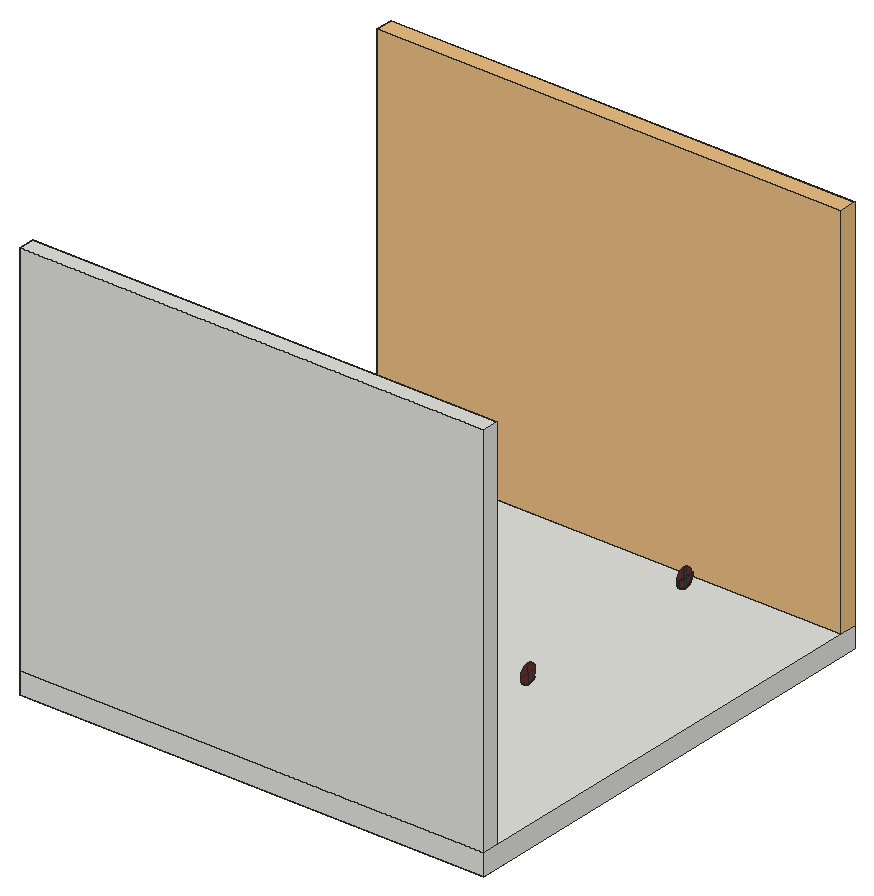
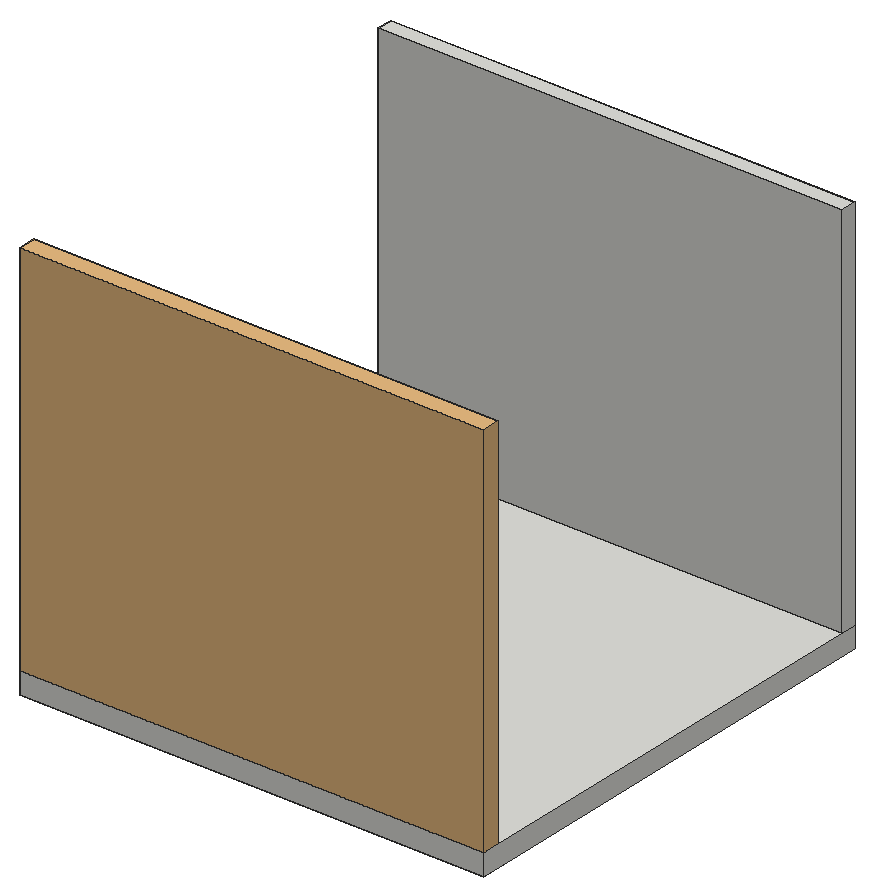
# SketchUp Ruby script. Lengths in millimetres.
U = 1.mm
M = Sketchup.active_model
def pt(a) = Geom::Point3d.new(a.map { |v| v * U })
def face(e, loops, mat)
  f = e.add_face(loops[0].map { |a| pt(a) })
  loops[1..].each { |l| e.add_face(l.map { |a| pt(a) }).erase! }
  f.material = f.back_material = mat if mat
  f
end
# faces: each face lists its corners as indices into pts; further lists are holes
def faces(e, pts, list, mat = nil) = list.each { |f| face(e, (f[0].is_a?(Array) ? f : [f]).map { |l| l.map { |i| pts[i] } }, mat) }
# xy, xz, yz: faces in a plane at the given z, y or x. An outline is a flat list of corners, or four numbers for a rectangle; further outlines are holes
def ring(l) = l.size == 4 ? [[l[0], l[1]], [l[2], l[1]], [l[2], l[3]], [l[0], l[3]]] : l.each_slice(2).to_a
def flat(e, list, mat, &to3) = list.each { |f| face(e, (f[0].is_a?(Array) ? f : [f]).map { |l| ring(l).map { |u, v| to3.(u, v) } }, mat) }
def xy(e, z, list, mat = nil) = flat(e, list, mat) { |x, y| [x, y, z] }
def xz(e, y, list, mat = nil) = flat(e, list, mat) { |x, z| [x, y, z] }
def yz(e, x, list, mat = nil) = flat(e, list, mat) { |y, z| [x, y, z] }
def lines(e, pts, list) = list.each { |a, b| e.add_line(pt(pts[a]), pt(pts[b])) }
# prism: a flat outline (further loops are holes) pulled along v
def prism(e, loops, v, mat = nil)
  f = face(e, loops, mat); d = Geom::Vector3d.new(v.map { |x| x * U })
  f.pushpull(f.normal.samedirection?(d) ? d.length : -d.length)
end
def box(e, o, s, mat = nil) = prism(e, [[o, [o[0] + s[0], o[1], o[2]], [o[0] + s[0], o[1] + s[1], o[2]], [o[0], o[1] + s[1], o[2]]]], [0, 0, s[2]], mat)
def at(x, y, z, deg = 0) = Geom::Transformation.translation(pt([x, y, z])) * Geom::Transformation.rotation(ORIGIN, Z_AXIS, deg.degrees)
def axes(o, x, y, z) = Geom::Transformation.new([*x, 0, *y, 0, *z, 0, *pt(o).to_a, 1])
def part(name) = M.definitions.add(name)
# library, detail: a bought-in or finely detailed component or shape, given as its bounding box
def library(name, o, s) = part(name).tap { |d| box(d.entities, o, s) }
def detail(e, o, s) = box(e.add_group.entities, o, s)
def put(e, d, t, mat = nil) = e.add_instance(d, t).tap { |i| i.material = mat if mat }
def group(e, t, mat = nil) = e.add_group.tap { |g| g.transformation = t; g.material = mat if mat }.entities
root = M.entities
M.materials.add("Uniboard-L17-Ambrette-4K").color = [104, 52, 49]
M.materials.add("Uniboard-L19-Putty-4K").color = [187, 181, 160]
c1 = library("Group\#2",[0,-12,0],[3352.8,126.3,2743.2])
xy(root,413.1,[[2619.9,1332.9,2628.9,1333.4],[2619.9,1336.4,2628.9,1336.9],[2616.9,2747.3,2628.9,2747.8],[2616.9,2750.8,2628.9,2751.3]],"Uniboard-L17-Ambrette-4K")
xy(root,478.1,[[2616.9,2684.3,2628.9,2747.8],[2616.9,2750.8,2628.9,2814.3]],"Uniboard-L17-Ambrette-4K")
xy(root,481.1,[[2616.9,2684.3,2628.9,2747.8],[2616.9,2750.8,2628.9,2814.3]],"Uniboard-L17-Ambrette-4K")
xz(root,2684.3,[[2616.9,476.1,2628.9,478.1],[2616.9,481.1,2628.9,483.1]],"Uniboard-L17-Ambrette-4K")
xz(root,2747.8,[[2616.9,413.1,2628.9,478.1],[2616.9,481.1,2628.9,546.1]],"Uniboard-L17-Ambrette-4K")
xz(root,2750.8,[[2616.9,413.1,2628.9,478.1],[2616.9,481.1,2628.9,546.1]],"Uniboard-L17-Ambrette-4K")
xz(root,2814.3,[[2616.9,476.1,2628.9,478.1],[2616.9,481.1,2628.9,483.1]],"Uniboard-L17-Ambrette-4K")
yz(root,2616.9,[[2747.3,413.1,2745.2,413.2,2741.2,413.6,2739.1,413.9,2733.1,415.1,2731.2,415.7,2729.2,416.3,2727.3,416.9,2725.4,417.7,2723.5,418.4,2721.6,419.3,2718,421.1,2716.2,422.2,2714.5,423.2,2712.8,424.3,2711.1,425.5,2709.5,426.7,2706.3,429.3,2703.3,432.1,2700.5,435.1,2697.9,438.3,2696.7,439.9,2695.5,441.6,2694.4,443.3,2693.4,445,2692.3,446.8,2690.5,450.4,2688.1,456.1,2687.5,458,2686.9,460,2686.3,461.9,2685.1,467.9,2684.8,470,2684.4,474,2684.3,476.1,2684.3,478.1,2747.8,478.1,2747.8,413.1],[2750.8,413.1,2750.8,478.1,2814.3,478.1,2814.3,476.1,2814.2,474,2813.8,470,2813.5,467.9,2813.2,465.9,2812.7,463.9,2812.3,461.9,2811.7,460,2811.1,458,2810.5,456.1,2809.7,454.2,2809,452.3,2808.1,450.4,2806.3,446.8,2805.3,445,2803.1,441.6,2801.9,439.9,2800.7,438.3,2798.1,435.1,2795.3,432.1,2792.3,429.3,2789.1,426.7,2787.5,425.5,2785.8,424.3,2784.1,423.2,2782.4,422.2,2780.6,421.1,2777,419.3,2775.1,418.4,2773.2,417.7,2771.3,416.9,2769.4,416.3,2767.4,415.7,2765.5,415.1,2759.5,413.9,2757.5,413.6,2755.4,413.4,2753.4,413.2,2751.3,413.1],[2684.3,481.1,2684.3,483.1,2684.4,485.2,2684.8,489.2,2685.1,491.3,2686.3,497.3,2686.9,499.2,2687.5,501.2,2688.1,503.1,2690.5,508.8,2692.3,512.4,2693.4,514.2,2694.4,515.9,2695.5,517.6,2696.7,519.3,2697.9,520.9,2700.5,524.1,2703.3,527.1,2706.3,529.9,2709.5,532.5,2711.1,533.7,2712.8,534.9,2714.5,536,2716.2,537,2718,538.1,2721.6,539.9,2723.5,540.8,2725.4,541.5,2727.3,542.3,2729.2,542.9,2731.2,543.5,2733.1,544.1,2739.1,545.3,2741.2,545.6,2745.2,546,2747.3,546.1,2747.8,546.1,2747.8,481.1],[2750.8,481.1,2750.8,546.1,2751.3,546.1,2753.4,546,2755.4,545.8,2757.5,545.6,2759.5,545.3,2765.5,544.1,2767.4,543.5,2769.4,542.9,2771.3,542.3,2773.2,541.5,2775.1,540.8,2777,539.9,2780.6,538.1,2782.4,537,2784.1,536,2785.8,534.9,2787.5,533.7,2789.1,532.5,2792.3,529.9,2795.3,527.1,2798.1,524.1,2800.7,520.9,2801.9,519.3,2803.1,517.6,2805.3,514.2,2806.3,512.4,2808.1,508.8,2809,506.9,2809.7,505,2810.5,503.1,2811.1,501.2,2811.7,499.2,2812.3,497.3,2812.7,495.3,2813.2,493.3,2813.5,491.3,2813.8,489.2,2814.2,485.2,2814.3,483.1,2814.3,481.1]],"Uniboard-L17-Ambrette-4K")
yz(root,2619.9,[[1332.9,413.1,1330.8,413.2,1326.8,413.6,1324.7,413.9,1318.7,415.1,1316.8,415.7,1314.8,416.3,1312.9,416.9,1311,417.7,1309.1,418.4,1307.2,419.3,1303.6,421.1,1301.8,422.2,1300.1,423.2,1298.4,424.3,1296.7,425.5,1295.1,426.7,1291.9,429.3,1288.9,432.1,1286.1,435.1,1283.5,438.3,1282.3,439.9,1281.1,441.6,1280,443.3,1279,445,1277.9,446.8,1276.1,450.4,1273.7,456.1,1273.1,458,1272.5,460,1271.9,461.9,1270.7,467.9,1270.4,470,1270,474,1269.9,476.1,1269.9,478.1,1333.4,478.1,1333.4,413.1],[1336.4,413.1,1336.4,478.1,1399.9,478.1,1399.9,476.1,1399.8,474,1399.4,470,1399.1,467.9,1398.8,465.9,1398.3,463.9,1397.9,461.9,1397.3,460,1396.7,458,1396.1,456.1,1395.3,454.2,1394.6,452.3,1393.7,450.4,1391.9,446.8,1390.9,445,1388.7,441.6,1387.5,439.9,1386.3,438.3,1383.7,435.1,1380.9,432.1,1377.9,429.3,1374.7,426.7,1373.1,425.5,1371.4,424.3,1369.7,423.2,1368,422.2,1366.2,421.1,1362.6,419.3,1360.7,418.4,1358.8,417.7,1356.9,416.9,1355,416.3,1353,415.7,1351.1,415.1,1345.1,413.9,1343.1,413.6,1341,413.4,1339,413.2,1336.9,413.1],[1269.9,481.1,1269.9,483.1,1270,485.2,1270.4,489.2,1270.7,491.3,1271.9,497.3,1272.5,499.2,1273.1,501.2,1273.7,503.1,1276.1,508.8,1277.9,512.4,1279,514.2,1280,515.9,1281.1,517.6,1282.3,519.3,1283.5,520.9,1286.1,524.1,1288.9,527.1,1291.9,529.9,1295.1,532.5,1296.7,533.7,1298.4,534.9,1300.1,536,1301.8,537,1303.6,538.1,1307.2,539.9,1309.1,540.8,1311,541.5,1312.9,542.3,1314.8,542.9,1316.8,543.5,1318.7,544.1,1324.7,545.3,1326.8,545.6,1330.8,546,1332.9,546.1,1333.4,546.1,1333.4,481.1],[1336.4,481.1,1336.4,546.1,1336.9,546.1,1339,546,1341,545.8,1343.1,545.6,1345.1,545.3,1351.1,544.1,1353,543.5,1355,542.9,1356.9,542.3,1358.8,541.5,1360.7,540.8,1362.6,539.9,1366.2,538.1,1368,537,1369.7,536,1371.4,534.9,1373.1,533.7,1374.7,532.5,1377.9,529.9,1380.9,527.1,1383.7,524.1,1386.3,520.9,1387.5,519.3,1388.7,517.6,1390.9,514.2,1391.9,512.4,1393.7,508.8,1394.6,506.9,1395.3,505,1396.1,503.1,1396.7,501.2,1397.3,499.2,1397.9,497.3,1398.3,495.3,1398.8,493.3,1399.1,491.3,1399.4,489.2,1399.8,485.2,1399.9,483.1,1399.9,481.1]],"Uniboard-L17-Ambrette-4K")
p = [[2628.9,1332.9,413.1],[2628.9,1330.8,413.2],[2619.9,1330.8,413.2],[2619.9,1332.9,413.1],[2628.9,1339,413.2],[2628.9,1336.9,413.1],
  [2619.9,1336.9,413.1],[2619.9,1339,413.2],[2628.9,2747.3,413.1],[2628.9,2745.2,413.2],[2616.9,2745.2,413.2],[2616.9,2747.3,413.1],
  [2628.9,2753.4,413.2],[2628.9,2751.3,413.1],[2616.9,2751.3,413.1],[2616.9,2753.4,413.2],[2628.9,1328.8,413.4],[2619.9,1328.8,413.4],
  [2628.9,1341,413.4],[2619.9,1341,413.4],[2628.9,2743.2,413.4],[2616.9,2743.2,413.4],[2628.9,2755.4,413.4],[2616.9,2755.4,413.4],
  [2628.9,1326.8,413.6],[2619.9,1326.8,413.6],[2628.9,1343.1,413.6],[2619.9,1343.1,413.6],[2628.9,2741.2,413.6],[2616.9,2741.2,413.6],
  [2628.9,2757.5,413.6],[2616.9,2757.5,413.6],[2628.9,1324.7,413.9],[2619.9,1324.7,413.9],[2628.9,1345.1,413.9],[2619.9,1345.1,413.9],
  [2628.9,2739.1,413.9],[2616.9,2739.1,413.9],[2628.9,2759.5,413.9],[2616.9,2759.5,413.9],[2628.9,1322.7,414.3],[2619.9,1322.7,414.3],
  [2628.9,1347.1,414.3],[2619.9,1347.1,414.3],[2628.9,2737.1,414.3],[2616.9,2737.1,414.3],[2628.9,2761.5,414.3],[2616.9,2761.5,414.3],
  [2628.9,1320.7,414.7],[2619.9,1320.7,414.7],[2628.9,1349.1,414.7],[2619.9,1349.1,414.7],[2628.9,2735.1,414.7],[2616.9,2735.1,414.7],
  [2628.9,2763.5,414.7],[2616.9,2763.5,414.7],[2628.9,1318.7,415.1],[2619.9,1318.7,415.1],[2628.9,1351.1,415.1],[2619.9,1351.1,415.1],
  [2628.9,2733.1,415.1],[2616.9,2733.1,415.1],[2628.9,2765.5,415.1],[2616.9,2765.5,415.1],[2628.9,1316.8,415.7],[2619.9,1316.8,415.7],
  [2628.9,1353,415.7],[2619.9,1353,415.7],[2628.9,2731.2,415.7],[2616.9,2731.2,415.7],[2628.9,2767.4,415.7],[2616.9,2767.4,415.7],
  [2628.9,1314.8,416.3],[2619.9,1314.8,416.3],[2628.9,1355,416.3],[2619.9,1355,416.3],[2628.9,2729.2,416.3],[2616.9,2729.2,416.3],
  [2628.9,2769.4,416.3],[2616.9,2769.4,416.3],[2628.9,1312.9,416.9],[2619.9,1312.9,416.9],[2628.9,1356.9,416.9],[2619.9,1356.9,416.9],
  [2628.9,2727.3,416.9],[2616.9,2727.3,416.9],[2628.9,2771.3,416.9],[2616.9,2771.3,416.9],[2628.9,1311,417.7],[2619.9,1311,417.7],
  [2628.9,1358.8,417.7],[2619.9,1358.8,417.7],[2628.9,2725.4,417.7],[2616.9,2725.4,417.7],[2628.9,2773.2,417.7],[2616.9,2773.2,417.7],
  [2628.9,1309.1,418.4],[2619.9,1309.1,418.4],[2628.9,1360.7,418.4],[2619.9,1360.7,418.4],[2628.9,2723.5,418.4],[2616.9,2723.5,418.4],
  [2628.9,2775.1,418.4],[2616.9,2775.1,418.4],[2628.9,1307.2,419.3],[2619.9,1307.2,419.3],[2628.9,1362.6,419.3],[2619.9,1362.6,419.3],
  [2628.9,2721.6,419.3],[2616.9,2721.6,419.3],[2628.9,2777,419.3],[2616.9,2777,419.3],[2628.9,1305.4,420.2],[2619.9,1305.4,420.2],
  [2628.9,1364.4,420.2],[2619.9,1364.4,420.2],[2628.9,2719.8,420.2],[2616.9,2719.8,420.2],[2628.9,2778.8,420.2],[2616.9,2778.8,420.2],
  [2628.9,1303.6,421.1],[2619.9,1303.6,421.1],[2628.9,1366.2,421.1],[2619.9,1366.2,421.1],[2628.9,2718,421.1],[2616.9,2718,421.1],
  [2628.9,2780.6,421.1],[2616.9,2780.6,421.1],[2628.9,1301.8,422.2],[2619.9,1301.8,422.2],[2628.9,1368,422.2],[2619.9,1368,422.2],
  [2628.9,2716.2,422.2],[2616.9,2716.2,422.2],[2628.9,2782.4,422.2],[2616.9,2782.4,422.2],[2628.9,1300.1,423.2],[2619.9,1300.1,423.2],
  [2628.9,1369.7,423.2],[2619.9,1369.7,423.2],[2628.9,2714.5,423.2],[2616.9,2714.5,423.2],[2628.9,2784.1,423.2],[2616.9,2784.1,423.2],
  [2628.9,1298.4,424.3],[2619.9,1298.4,424.3],[2628.9,1371.4,424.3],[2619.9,1371.4,424.3],[2628.9,2712.8,424.3],[2616.9,2712.8,424.3],
  [2628.9,2785.8,424.3],[2616.9,2785.8,424.3],[2628.9,1296.7,425.5],[2619.9,1296.7,425.5],[2628.9,1373.1,425.5],[2619.9,1373.1,425.5],
  [2628.9,2711.1,425.5],[2616.9,2711.1,425.5],[2628.9,2787.5,425.5],[2616.9,2787.5,425.5],[2628.9,1295.1,426.7],[2619.9,1295.1,426.7],
  [2628.9,1374.7,426.7],[2619.9,1374.7,426.7],[2628.9,2709.5,426.7],[2616.9,2709.5,426.7],[2628.9,2789.1,426.7],[2616.9,2789.1,426.7],
  [2628.9,1293.5,428],[2619.9,1293.5,428],[2628.9,1376.3,428],[2619.9,1376.3,428],[2628.9,2707.9,428],[2616.9,2707.9,428],
  [2628.9,2790.7,428],[2616.9,2790.7,428],[2628.9,1291.9,429.3],[2619.9,1291.9,429.3],[2628.9,1377.9,429.3],[2619.9,1377.9,429.3],
  [2628.9,2706.3,429.3],[2616.9,2706.3,429.3],[2628.9,2792.3,429.3],[2616.9,2792.3,429.3],[2628.9,1290.4,430.7],[2619.9,1290.4,430.7],
  [2628.9,1379.4,430.7],[2619.9,1379.4,430.7],[2628.9,2704.8,430.7],[2616.9,2704.8,430.7],[2628.9,2793.8,430.7],[2616.9,2793.8,430.7],
  [2628.9,1288.9,432.1],[2619.9,1288.9,432.1],[2628.9,1380.9,432.1],[2619.9,1380.9,432.1],[2628.9,2703.3,432.1],[2616.9,2703.3,432.1],
  [2628.9,2795.3,432.1],[2616.9,2795.3,432.1],[2628.9,1287.5,433.6],[2619.9,1287.5,433.6],[2628.9,1382.3,433.6],[2619.9,1382.3,433.6],
  [2628.9,2701.9,433.6],[2616.9,2701.9,433.6],[2628.9,2796.7,433.6],[2616.9,2796.7,433.6],[2628.9,1286.1,435.1],[2619.9,1286.1,435.1],
  [2628.9,1383.7,435.1],[2619.9,1383.7,435.1],[2628.9,2700.5,435.1],[2616.9,2700.5,435.1],[2628.9,2798.1,435.1],[2616.9,2798.1,435.1],
  [2628.9,1284.8,436.7],[2619.9,1284.8,436.7],[2628.9,1385,436.7],[2619.9,1385,436.7],[2628.9,2699.2,436.7],[2616.9,2699.2,436.7],
  [2628.9,2799.4,436.7],[2616.9,2799.4,436.7],[2628.9,1283.5,438.3],[2619.9,1283.5,438.3],[2628.9,1386.3,438.3],[2619.9,1386.3,438.3],
  [2628.9,2697.9,438.3],[2616.9,2697.9,438.3],[2628.9,2800.7,438.3],[2616.9,2800.7,438.3],[2628.9,2696.7,439.9],[2616.9,2696.7,439.9],
  [2628.9,2801.9,439.9],[2616.9,2801.9,439.9],[2628.9,2695.5,441.6],[2616.9,2695.5,441.6],[2628.9,2803.1,441.6],[2616.9,2803.1,441.6],
  [2628.9,2694.4,443.3],[2616.9,2694.4,443.3],[2628.9,2804.2,443.3],[2616.9,2804.2,443.3],[2628.9,2693.4,445],[2616.9,2693.4,445],
  [2628.9,2805.3,445],[2616.9,2805.3,445],[2628.9,2692.3,446.8],[2616.9,2692.3,446.8],[2628.9,2806.3,446.8],[2616.9,2806.3,446.8],
  [2628.9,2691.4,448.6],[2616.9,2691.4,448.6],[2628.9,2807.2,448.6],[2616.9,2807.2,448.6],[2628.9,2690.5,450.4],[2616.9,2690.5,450.4],
  [2628.9,2808.1,450.4],[2616.9,2808.1,450.4],[2628.9,2689.7,452.3],[2616.9,2689.7,452.3],[2628.9,2809,452.3],[2616.9,2809,452.3],
  [2628.9,2688.9,454.2],[2616.9,2688.9,454.2],[2628.9,2809.7,454.2],[2616.9,2809.7,454.2],[2628.9,2688.1,456.1],[2616.9,2688.1,456.1],
  [2628.9,2810.5,456.1],[2616.9,2810.5,456.1],[2628.9,2687.5,458],[2616.9,2687.5,458],[2628.9,2811.1,458],[2616.9,2811.1,458],
  [2628.9,2686.9,460],[2616.9,2686.9,460],[2628.9,2811.7,460],[2616.9,2811.7,460],[2628.9,2686.3,461.9],[2616.9,2686.3,461.9],
  [2628.9,2812.3,461.9],[2616.9,2812.3,461.9],[2628.9,2685.9,463.9],[2616.9,2685.9,463.9],[2628.9,2812.7,463.9],[2616.9,2812.7,463.9],
  [2628.9,2685.5,465.9],[2616.9,2685.5,465.9],[2628.9,2813.2,465.9],[2616.9,2813.2,465.9],[2628.9,2685.1,467.9],[2616.9,2685.1,467.9],
  [2628.9,2813.5,467.9],[2616.9,2813.5,467.9],[2628.9,2684.8,470],[2616.9,2684.8,470],[2628.9,2813.8,470],[2616.9,2813.8,470],
  [2628.9,2684.6,472],[2616.9,2684.6,472],[2628.9,2814,472],[2616.9,2814,472],[2628.9,2684.4,474],[2616.9,2684.4,474],
  [2628.9,2814.2,474],[2616.9,2814.2,474],[2628.9,2684.3,476.1],[2616.9,2684.3,476.1],[2628.9,2814.3,476.1],[2616.9,2814.3,476.1],
  [2628.9,2684.3,483.1],[2628.9,2684.4,485.2],[2616.9,2684.4,485.2],[2616.9,2684.3,483.1],[2628.9,2814.2,485.2],[2628.9,2814.3,483.1],
  [2616.9,2814.3,483.1],[2616.9,2814.2,485.2],[2628.9,2684.6,487.2],[2616.9,2684.6,487.2],[2628.9,2814,487.2],[2616.9,2814,487.2],
  [2628.9,2684.8,489.2],[2616.9,2684.8,489.2],[2628.9,2813.8,489.2],[2616.9,2813.8,489.2]]
faces(root,p,[[0,1,2,3],[4,5,6,7],[8,9,10,11],[12,13,14,15],[1,16,17,2],[18,4,7,19],[9,20,21,10],[22,12,15,23],
  [16,24,25,17],[26,18,19,27],[20,28,29,21],[30,22,23,31],[24,32,33,25],[34,26,27,35],[28,36,37,29],[38,30,31,39],
  [32,40,41,33],[42,34,35,43],[36,44,45,37],[46,38,39,47],[40,48,49,41],[50,42,43,51],[44,52,53,45],[54,46,47,55],
  [48,56,57,49],[58,50,51,59],[52,60,61,53],[62,54,55,63],[56,64,65,57],[66,58,59,67],[60,68,69,61],[70,62,63,71],
  [64,72,73,65],[74,66,67,75],[68,76,77,69],[78,70,71,79],[72,80,81,73],[82,74,75,83],[76,84,85,77],[86,78,79,87],
  [80,88,89,81],[90,82,83,91],[84,92,93,85],[94,86,87,95],[88,96,97,89],[98,90,91,99],[92,100,101,93],[102,94,95,103],
  [96,104,105,97],[106,98,99,107],[100,108,109,101],[110,102,103,111],[104,112,113,105],[114,106,107,115],[108,116,117,109],[118,110,111,119],
  [112,120,121,113],[122,114,115,123],[116,124,125,117],[126,118,119,127],[120,128,129,121],[130,122,123,131],[124,132,133,125],[134,126,127,135],
  [128,136,137,129],[138,130,131,139],[132,140,141,133],[142,134,135,143],[136,144,145,137],[146,138,139,147],[140,148,149,141],[150,142,143,151],
  [144,152,153,145],[154,146,147,155],[148,156,157,149],[158,150,151,159],[152,160,161,153],[162,154,155,163],[156,164,165,157],[166,158,159,167],
  [160,168,169,161],[170,162,163,171],[164,172,173,165],[174,166,167,175],[168,176,177,169],[178,170,171,179],[172,180,181,173],[182,174,175,183],
  [176,184,185,177],[186,178,179,187],[180,188,189,181],[190,182,183,191],[184,192,193,185],[194,186,187,195],[188,196,197,189],[198,190,191,199],
  [192,200,201,193],[202,194,195,203],[196,204,205,197],[206,198,199,207],[200,208,209,201],[210,202,203,211],[204,212,213,205],[214,206,207,215],
  [208,216,217,209],[218,210,211,219],[212,220,221,213],[222,214,215,223],[216,224,225,217],[226,218,219,227],[220,228,229,221],[230,222,223,231],
  [228,232,233,229],[234,230,231,235],[232,236,237,233],[238,234,235,239],[236,240,241,237],[242,238,239,243],[240,244,245,241],[246,242,243,247],
  [244,248,249,245],[250,246,247,251],[248,252,253,249],[254,250,251,255],[252,256,257,253],[258,254,255,259],[256,260,261,257],[262,258,259,263],
  [260,264,265,261],[266,262,263,267],[264,268,269,265],[270,266,267,271],[268,272,273,269],[274,270,271,275],[272,276,277,273],[278,274,275,279],
  [276,280,281,277],[282,278,279,283],[280,284,285,281],[286,282,283,287],[284,288,289,285],[290,286,287,291],[288,292,293,289],[294,290,291,295],
  [292,296,297,293],[298,294,295,299],[296,300,301,297],[302,298,299,303],[300,304,305,301],[306,302,303,307],[304,308,309,305],[310,306,307,311],
  [312,313,314,315],[316,317,318,319],[313,320,321,314],[322,316,319,323],[320,324,325,321],[326,322,323,327]],"Uniboard-L17-Ambrette-4K")
g1 = group(root,at(0,20.3,0))
box(g1,[0,0,0],[3352.8,3352.8,152.4])
put(root,c1,at(0,3258.8,152.4),"Uniboard-L19-Putty-4K")
g2 = group(root,at(0,20.3,152.4))
box(g2,[0,0,0],[3352.8,114.3,2743.2])
